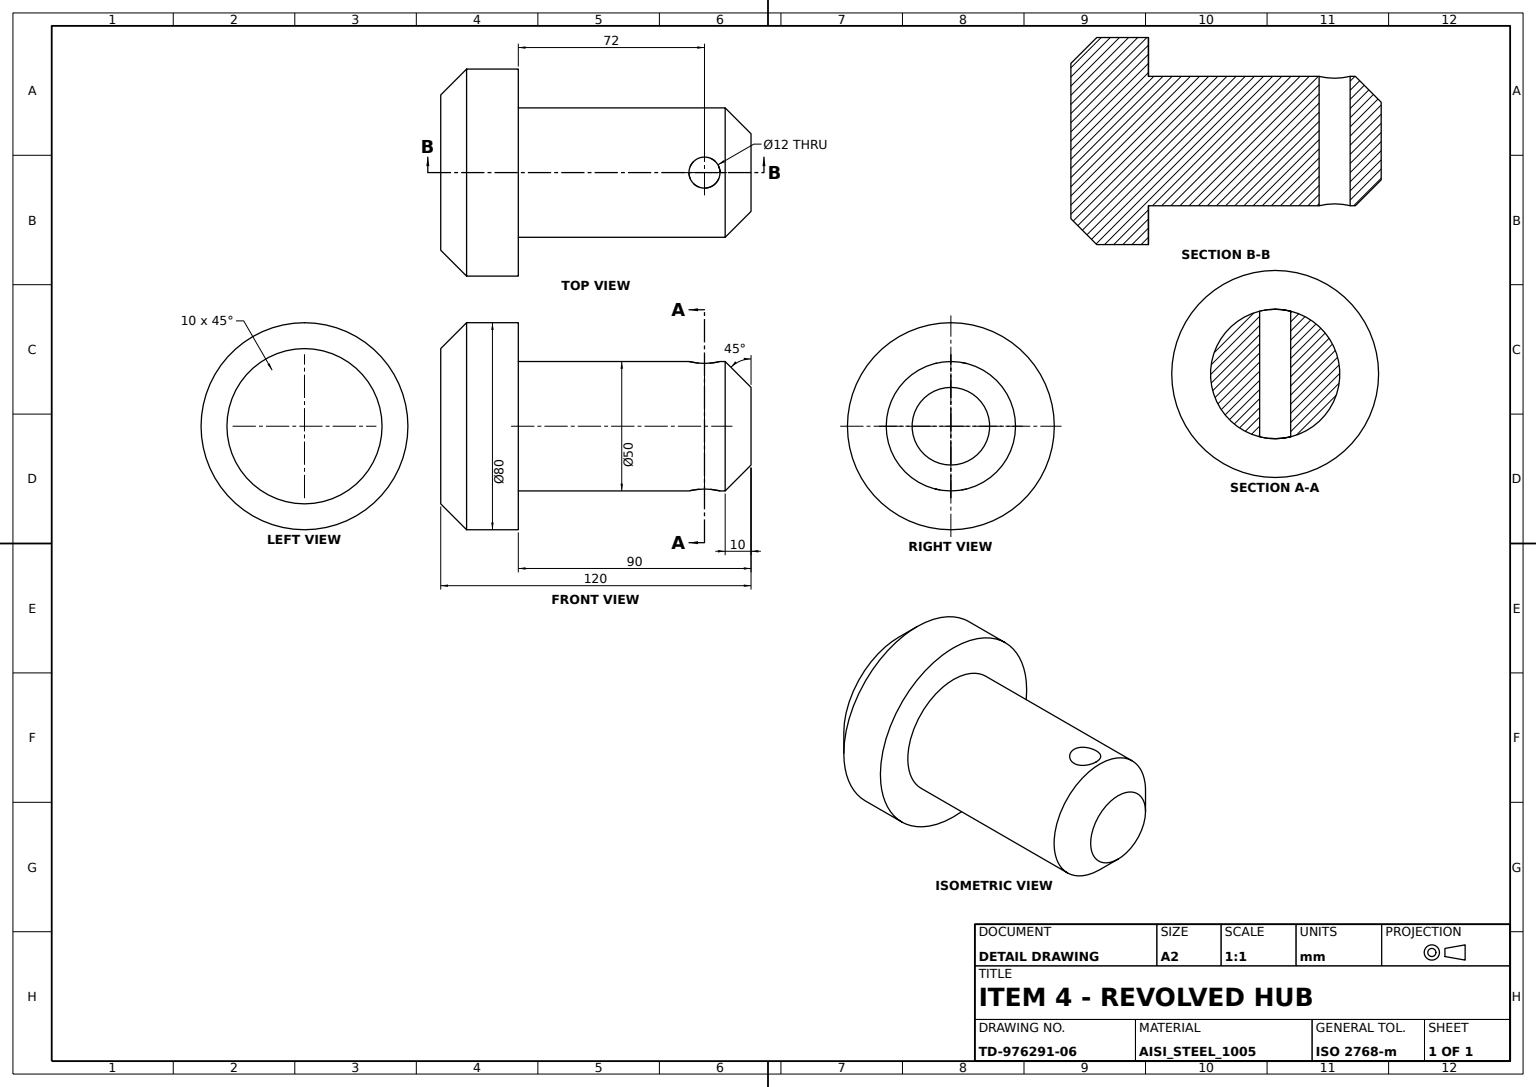
ISO-10303-21;
HEADER;
FILE_DESCRIPTION((''),'2;1');
FILE_NAME('','',(''),(''),'','','');
FILE_SCHEMA(('AUTOMOTIVE_DESIGN'));
ENDSEC;
DATA;
#1=APPLICATION_CONTEXT('');
#2=PRODUCT_CONTEXT('',#1,'mechanical');
#3=PRODUCT('','','',(#2));
#4=PRODUCT_DEFINITION_FORMATION('','',#3);
#5=PRODUCT_DEFINITION_CONTEXT('',#1,'design');
#6=PRODUCT_DEFINITION('','',#4,#5);
#7=PRODUCT_DEFINITION_SHAPE('','',#6);
#8=(LENGTH_UNIT()NAMED_UNIT(*)SI_UNIT(.MILLI.,.METRE.));
#9=(NAMED_UNIT(*)PLANE_ANGLE_UNIT()SI_UNIT($,.RADIAN.));
#10=(NAMED_UNIT(*)SI_UNIT($,.STERADIAN.)SOLID_ANGLE_UNIT());
#11=UNCERTAINTY_MEASURE_WITH_UNIT(LENGTH_MEASURE(0.005),#8,'distance_accuracy_value','');
#12=(GEOMETRIC_REPRESENTATION_CONTEXT(3)GLOBAL_UNCERTAINTY_ASSIGNED_CONTEXT((#11))GLOBAL_UNIT_ASSIGNED_CONTEXT((#8,#9,#10))REPRESENTATION_CONTEXT('',''));
#13=CARTESIAN_POINT('',(110.,0.,25.));
#14=VERTEX_POINT('',#13);
#15=CARTESIAN_POINT('',(110.,0.,0.));
#16=DIRECTION('',(-1.,0.,0.));
#17=DIRECTION('',(0.,0.,1.));
#18=AXIS2_PLACEMENT_3D('',#15,#16,#17);
#19=CIRCLE('',#18,25.);
#20=EDGE_CURVE('',#14,#14,#19,.T.);
#21=ORIENTED_EDGE('',*,*,#20,.F.);
#22=EDGE_LOOP('',(#21));
#23=FACE_BOUND('',#22,.T.);
#24=CARTESIAN_POINT('',(120.,0.,15.));
#25=VERTEX_POINT('',#24);
#26=CARTESIAN_POINT('',(120.,0.,0.));
#27=AXIS2_PLACEMENT_3D('',#26,#16,#17);
#28=CIRCLE('',#27,15.);
#29=EDGE_CURVE('',#25,#25,#28,.T.);
#30=ORIENTED_EDGE('',*,*,#29,.T.);
#31=EDGE_LOOP('',(#30));
#32=FACE_BOUND('',#31,.T.);
#33=CONICAL_SURFACE('',#27,15.,0.785398163);
#34=ADVANCED_FACE('',(#23,#32),#33,.T.);
#35=ORIENTED_EDGE('',*,*,#29,.F.);
#36=EDGE_LOOP('',(#35));
#37=FACE_BOUND('',#36,.T.);
#38=PLANE('',#27);
#39=ADVANCED_FACE('',(#37),#38,.F.);
#40=CARTESIAN_POINT('',(30.,0.,25.));
#41=VERTEX_POINT('',#40);
#42=CARTESIAN_POINT('',(30.,0.,0.));
#43=AXIS2_PLACEMENT_3D('',#42,#16,#17);
#44=CIRCLE('',#43,25.);
#45=EDGE_CURVE('',#41,#41,#44,.T.);
#46=ORIENTED_EDGE('',*,*,#45,.F.);
#47=EDGE_LOOP('',(#46));
#48=FACE_BOUND('',#47,.T.);
#49=CARTESIAN_POINT('',(96.,0.,-25.));
#50=VERTEX_POINT('',#49);
#51=CARTESIAN_POINT('',(96.318712,-2.372191,-24.92076));
#52=CARTESIAN_POINT('',(95.841192,0.001741,-25.039493));
#53=CARTESIAN_POINT('',(96.31652,2.365229,-24.921268));
#54=CARTESIAN_POINT('',(97.649263,4.352987,-24.637841));
#55=CARTESIAN_POINT('',(99.635345,5.683426,-24.350769));
#56=CARTESIAN_POINT('',(101.995582,6.15755,-24.228768));
#57=CARTESIAN_POINT('',(104.359883,5.686369,-24.350095));
#58=CARTESIAN_POINT('',(106.352196,4.352202,-24.638039));
#59=CARTESIAN_POINT('',(107.683992,2.363852,-24.92142));
#60=CARTESIAN_POINT('',(108.157511,0.002715,-25.039178));
#61=CARTESIAN_POINT('',(107.685962,-2.359581,-24.921868));
#62=CARTESIAN_POINT('',(106.355138,-4.348636,-24.638657));
#63=CARTESIAN_POINT('',(104.368604,-5.682431,-24.351043));
#64=CARTESIAN_POINT('',(102.003182,-6.157998,-24.228645));
#65=CARTESIAN_POINT('',(99.639016,-5.685572,-24.350311));
#66=CARTESIAN_POINT('',(97.65103,-4.35394,-24.637526));
#67=B_SPLINE_CURVE_WITH_KNOTS('',3,(#51,#52,#53,#54,#55,#56,#57,#58,#59,#60,#61,#62,#63,#64,#65,#66,#51,#52,#53),.UNSPECIFIED.,.T.,.F.,(1,1,1,1,1,1,1,1,1,1,1,1,1,1,1,1,1,1,1,1,1,1,1),(-0.007059428,-0.004706285,-0.002353143,0.,0.002353143,0.004706285,0.007059428,0.009412571,0.011765714,0.014118856,0.016471999,0.018825142,0.021178284,0.023531427,0.02588457,0.028237712,0.030590855,0.032943998,0.035297141,0.037650283,0.040003426,0.042356569,0.044709711),.UNSPECIFIED.);
#68=EDGE_CURVE('',#50,#50,#67,.T.);
#69=ORIENTED_EDGE('',*,*,#68,.F.);
#70=EDGE_LOOP('',(#69));
#71=FACE_BOUND('',#70,.T.);
#72=CARTESIAN_POINT('',(108.,0.,25.));
#73=VERTEX_POINT('',#72);
#74=CARTESIAN_POINT('',(107.681288,-2.372191,24.92076));
#75=CARTESIAN_POINT('',(108.158808,0.001741,25.039493));
#76=CARTESIAN_POINT('',(107.68348,2.365229,24.921268));
#77=CARTESIAN_POINT('',(106.350737,4.352987,24.637841));
#78=CARTESIAN_POINT('',(104.364655,5.683426,24.350769));
#79=CARTESIAN_POINT('',(102.004418,6.15755,24.228768));
#80=CARTESIAN_POINT('',(99.640117,5.686369,24.350095));
#81=CARTESIAN_POINT('',(97.647804,4.352202,24.638039));
#82=CARTESIAN_POINT('',(96.316008,2.363852,24.92142));
#83=CARTESIAN_POINT('',(95.842489,0.002715,25.039178));
#84=CARTESIAN_POINT('',(96.314038,-2.359581,24.921868));
#85=CARTESIAN_POINT('',(97.644862,-4.348636,24.638657));
#86=CARTESIAN_POINT('',(99.631396,-5.682431,24.351043));
#87=CARTESIAN_POINT('',(101.996818,-6.157998,24.228645));
#88=CARTESIAN_POINT('',(104.360984,-5.685572,24.350311));
#89=CARTESIAN_POINT('',(106.34897,-4.35394,24.637526));
#90=B_SPLINE_CURVE_WITH_KNOTS('',3,(#74,#75,#76,#77,#78,#79,#80,#81,#82,#83,#84,#85,#86,#87,#88,#89,#74,#75,#76),.UNSPECIFIED.,.T.,.F.,(1,1,1,1,1,1,1,1,1,1,1,1,1,1,1,1,1,1,1,1,1,1,1),(-0.007059428,-0.004706285,-0.002353143,0.,0.002353143,0.004706285,0.007059428,0.009412571,0.011765714,0.014118856,0.016471999,0.018825142,0.021178284,0.023531427,0.02588457,0.028237712,0.030590855,0.032943998,0.035297141,0.037650283,0.040003426,0.042356569,0.044709711),.UNSPECIFIED.);
#91=EDGE_CURVE('',#73,#73,#90,.T.);
#92=ORIENTED_EDGE('',*,*,#91,.F.);
#93=EDGE_LOOP('',(#92));
#94=FACE_BOUND('',#93,.T.);
#95=ORIENTED_EDGE('',*,*,#20,.T.);
#96=EDGE_LOOP('',(#95));
#97=FACE_BOUND('',#96,.T.);
#98=CARTESIAN_POINT('',(0.,0.,0.));
#99=AXIS2_PLACEMENT_3D('',#98,#16,#17);
#100=CYLINDRICAL_SURFACE('',#99,25.);
#101=ADVANCED_FACE('',(#48,#71,#94,#97),#100,.T.);
#102=CARTESIAN_POINT('',(0.,0.,30.));
#103=VERTEX_POINT('',#102);
#104=CIRCLE('',#99,30.);
#105=EDGE_CURVE('',#103,#103,#104,.T.);
#106=ORIENTED_EDGE('',*,*,#105,.F.);
#107=EDGE_LOOP('',(#106));
#108=FACE_BOUND('',#107,.T.);
#109=CARTESIAN_POINT('',(10.,0.,40.));
#110=VERTEX_POINT('',#109);
#111=CARTESIAN_POINT('',(10.,0.,0.));
#112=AXIS2_PLACEMENT_3D('',#111,#16,#17);
#113=CIRCLE('',#112,40.);
#114=EDGE_CURVE('',#110,#110,#113,.T.);
#115=ORIENTED_EDGE('',*,*,#114,.T.);
#116=EDGE_LOOP('',(#115));
#117=FACE_BOUND('',#116,.T.);
#118=DIRECTION('',(1.,0.,0.));
#119=DIRECTION('',(0.,0.,-1.));
#120=AXIS2_PLACEMENT_3D('',#111,#118,#119);
#121=CONICAL_SURFACE('',#120,40.,0.785398163);
#122=ADVANCED_FACE('',(#108,#117),#121,.T.);
#123=ORIENTED_EDGE('',*,*,#105,.T.);
#124=EDGE_LOOP('',(#123));
#125=FACE_BOUND('',#124,.T.);
#126=AXIS2_PLACEMENT_3D('',#102,#118,#119);
#127=PLANE('',#126);
#128=ADVANCED_FACE('',(#125),#127,.F.);
#129=CARTESIAN_POINT('',(30.,0.,40.));
#130=VERTEX_POINT('',#129);
#131=CIRCLE('',#43,40.);
#132=EDGE_CURVE('',#130,#130,#131,.T.);
#133=ORIENTED_EDGE('',*,*,#132,.F.);
#134=EDGE_LOOP('',(#133));
#135=FACE_BOUND('',#134,.T.);
#136=ORIENTED_EDGE('',*,*,#45,.T.);
#137=EDGE_LOOP('',(#136));
#138=FACE_BOUND('',#137,.T.);
#139=AXIS2_PLACEMENT_3D('',#40,#16,#17);
#140=PLANE('',#139);
#141=ADVANCED_FACE('',(#135,#138),#140,.F.);
#142=ORIENTED_EDGE('',*,*,#68,.T.);
#143=EDGE_LOOP('',(#142));
#144=FACE_BOUND('',#143,.T.);
#145=ORIENTED_EDGE('',*,*,#91,.T.);
#146=EDGE_LOOP('',(#145));
#147=FACE_BOUND('',#146,.T.);
#148=CARTESIAN_POINT('',(102.,0.,30.));
#149=AXIS2_PLACEMENT_3D('',#148,#119,#16);
#150=CYLINDRICAL_SURFACE('',#149,6.);
#151=ADVANCED_FACE('',(#144,#147),#150,.F.);
#152=ORIENTED_EDGE('',*,*,#114,.F.);
#153=EDGE_LOOP('',(#152));
#154=FACE_BOUND('',#153,.T.);
#155=ORIENTED_EDGE('',*,*,#132,.T.);
#156=EDGE_LOOP('',(#155));
#157=FACE_BOUND('',#156,.T.);
#158=CYLINDRICAL_SURFACE('',#99,40.);
#159=ADVANCED_FACE('',(#154,#157),#158,.T.);
#160=CLOSED_SHELL('',(#34,#39,#101,#122,#128,#141,#151,#159));
#161=MANIFOLD_SOLID_BREP('',#160);
#162=ADVANCED_BREP_SHAPE_REPRESENTATION('',(#161),#12);
#163=SHAPE_DEFINITION_REPRESENTATION(#7,#162);
ENDSEC;
END-ISO-10303-21;
